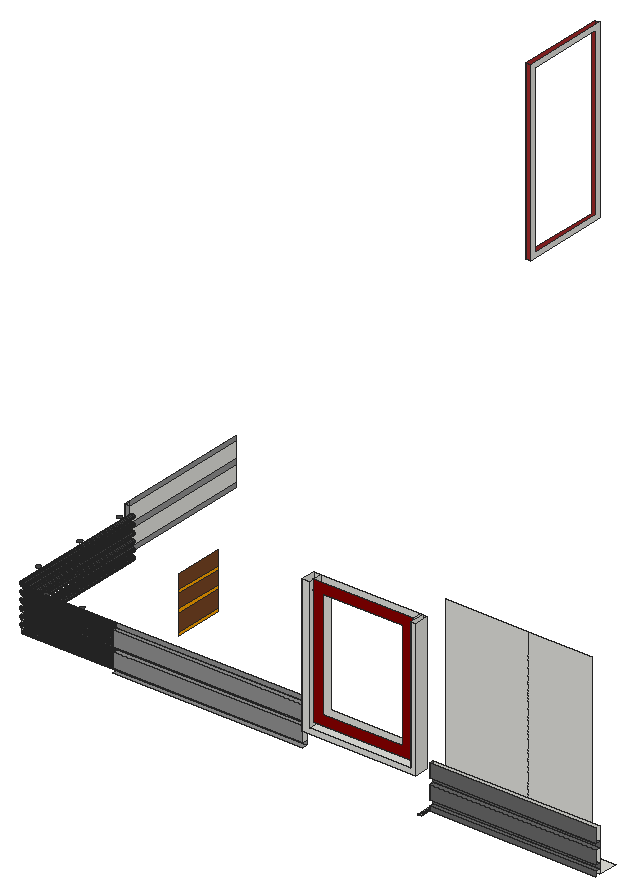
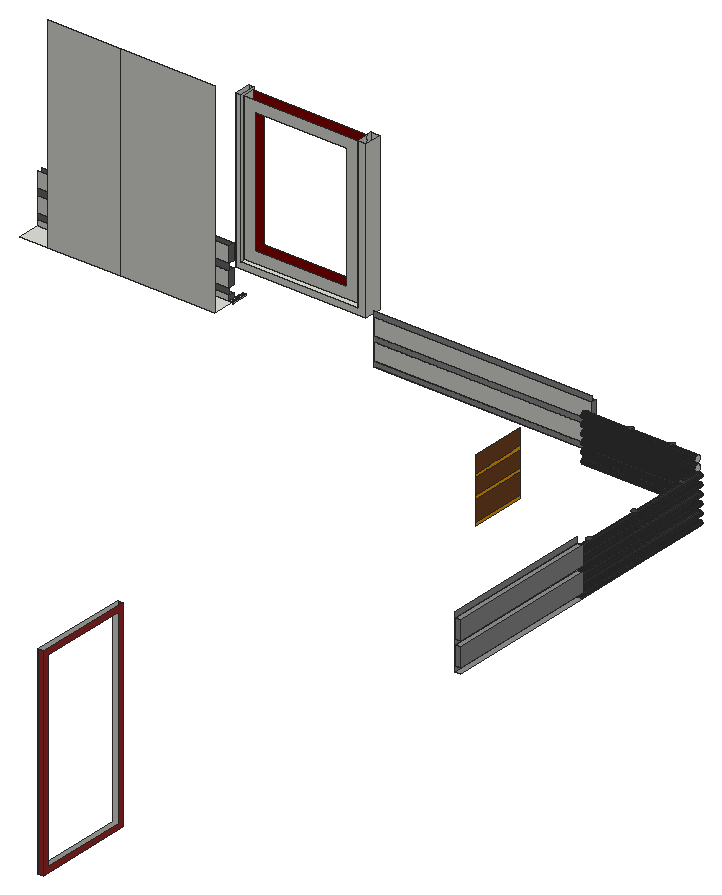
# SketchUp Ruby script. Lengths in inches.
U = 1.inch
M = Sketchup.active_model
def pt(a) = Geom::Point3d.new(a.map { |v| v * U })
def face(e, loops, mat)
  f = e.add_face(loops[0].map { |a| pt(a) })
  loops[1..].each { |l| e.add_face(l.map { |a| pt(a) }).erase! }
  f.material = f.back_material = mat if mat
  f
end
# faces: each face lists its corners as indices into pts; further lists are holes
def faces(e, pts, list, mat = nil) = list.each { |f| face(e, (f[0].is_a?(Array) ? f : [f]).map { |l| l.map { |i| pts[i] } }, mat) }
# xy, xz, yz: faces in a plane at the given z, y or x. An outline is a flat list of corners, or four numbers for a rectangle; further outlines are holes
def ring(l) = l.size == 4 ? [[l[0], l[1]], [l[2], l[1]], [l[2], l[3]], [l[0], l[3]]] : l.each_slice(2).to_a
def flat(e, list, mat, &to3) = list.each { |f| face(e, (f[0].is_a?(Array) ? f : [f]).map { |l| ring(l).map { |u, v| to3.(u, v) } }, mat) }
def xy(e, z, list, mat = nil) = flat(e, list, mat) { |x, y| [x, y, z] }
def xz(e, y, list, mat = nil) = flat(e, list, mat) { |x, z| [x, y, z] }
def yz(e, x, list, mat = nil) = flat(e, list, mat) { |y, z| [x, y, z] }
def lines(e, pts, list) = list.each { |a, b| e.add_line(pt(pts[a]), pt(pts[b])) }
# prism: a flat outline (further loops are holes) pulled along v
def prism(e, loops, v, mat = nil)
  f = face(e, loops, mat); d = Geom::Vector3d.new(v.map { |x| x * U })
  f.pushpull(f.normal.samedirection?(d) ? d.length : -d.length)
end
def box(e, o, s, mat = nil) = prism(e, [[o, [o[0] + s[0], o[1], o[2]], [o[0] + s[0], o[1] + s[1], o[2]], [o[0], o[1] + s[1], o[2]]]], [0, 0, s[2]], mat)
def at(x, y, z, deg = 0) = Geom::Transformation.translation(pt([x, y, z])) * Geom::Transformation.rotation(ORIGIN, Z_AXIS, deg.degrees)
def axes(o, x, y, z) = Geom::Transformation.new([*x, 0, *y, 0, *z, 0, *pt(o).to_a, 1])
def part(name) = M.definitions.add(name)
# library, detail: a bought-in or finely detailed component or shape, given as its bounding box
def library(name, o, s) = part(name).tap { |d| box(d.entities, o, s) }
def detail(e, o, s) = box(e.add_group.entities, o, s)
def put(e, d, t, mat = nil) = e.add_instance(d, t).tap { |i| i.material = mat if mat }
def group(e, t, mat = nil) = e.add_group.tap { |g| g.transformation = t; g.material = mat if mat }.entities
root = M.entities
M.materials.add("[0018_Brown]").color = [165, 42, 42]
M.materials.add("[0021_DarkRed]").color = [139, 0, 0]
M.materials.add("[0038_Orange]").color = [255, 165, 0]
M.materials.add("[0134_DimGray]").color = [105, 105, 105]
M.materials.add("[0137_Black]").color = [71, 71, 71]
M.materials.add("[Color M05]").color = [145, 145, 145]
M.materials.add("[Wood Veneer 01]").color = [120, 70, 37]
xy(root,247.03,[[8.875,116.75,11.875,199.5]],"[Color M05]")
xy(root,247.33,[[284.05,1.5,284.41,10.0625]])
xy(root,247.83,[[285.29,2.8125,286.17,10.0625]])
xy(root,247.89,[[284.05,1.0625,284.41,1.5],[284.41,1.0625,285.29,1.5625],[285.29,1.0625,286.17,2.8125],[284.05,1.5,284.41,10.0625],[284.41,1.5625,285.29,10.0625],
  [285.29,2.8125,286.17,10.0625],[286.17,7.0625,335.53,10.0625],[335.53,7.0625,375.29,10.0625],[284.41,10.0625,335.53,22.0625],[335.53,10.0625,390.0625,22.0625]])
xy(root,249.65,[[82.85,15.1875,200.79,18.1875]],"[Color M05]")
xy(root,250.07,[[8.875,116.75,11.875,199.5]],"[Color M05]")
xy(root,250.6875,[[286.17,7.0625,335.53,10.0625],[335.53,7.0625,390.0625,10.0625]],"[0134_DimGray]")
xy(root,252.55,[[82.85,15.1875,200.79,18.1875]])
xy(root,254.27,[[286.17,7.0625,390.0625,10.0625]],"[0134_DimGray]")
xy(root,260.15,[[8.875,116.75,11.875,199.5]],"[Color M05]")
xy(root,261.65,[[82.85,15.1875,200.79,18.1875]],"[Color M05]")
xy(root,262.6875,[[286.17,7.0625,390.0625,10.0625]],"[0134_DimGray]")
xy(root,263.19,[[8.875,116.75,11.875,199.5]],"[Color M05]")
xy(root,264.55,[[82.85,15.1875,200.79,18.1875]])
xy(root,266.27,[[286.17,7.0625,390.0625,10.0625]],"[0134_DimGray]")
xy(root,267.29,[[209.95,3.1875,280.75,12.1875]])
xy(root,270.55,[[214.5625,3.1875,278.01,12.1875]])
xy(root,271.42,[[12.37,43.72,12.71,43.74,13.04,43.84,13.33,44.02,13.56,44.27,13.72,44.58,13.79,44.91,13.78,45.25,13.68,45.58,13.49,45.87,13.24,46.1,12.9375,46.26,12.61,46.34,12.26,46.32,11.9375,46.22,11.65,46.04,11.41,45.79,11.25,45.48,11.18,45.15,11.19,44.81,11.29,44.48,11.48,44.1875,11.73,43.96,12.03,43.8],[12.37,75.91,12.71,75.92,13.04,76.03,13.33,76.21,13.56,76.46,13.72,76.76,13.79,77.1,13.78,77.44,13.68,77.77,13.49,78.06,13.24,78.29,12.9375,78.45,12.61,78.52,12.26,78.51,11.9375,78.41,11.65,78.23,11.41,77.97,11.25,77.67,11.18,77.34,11.19,76.99,11.29,76.67,11.48,76.375,11.73,76.14,12.03,75.99],[12.37,106.53,12.71,106.55,13.04,106.65,13.33,106.83,13.56,107.09,13.72,107.39,13.79,107.72,13.78,108.07,13.68,108.39,13.49,108.68,13.24,108.91,12.9375,109.07,12.61,109.15,12.26,109.14,11.9375,109.03,11.65,108.85,11.41,108.6,11.25,108.3,11.18,107.96,11.19,107.62,11.29,107.29,11.48,107,11.73,106.77,12.03,106.61]],"[0137_Black]")
xy(root,272.86,[[214.5625,6.1875,276.625,12.1875]])
xy(root,272.92,[[34.4,22.66,34.7,22.71,34.99,22.82,35.24,23.01,35.43,23.26,35.54,23.54,35.58,23.85,35.54,24.16,35.43,24.45,35.24,24.69,34.99,24.88,34.7,25,34.4,25.04,34.09,25,33.8,24.88,33.56,24.69,33.37,24.45,33.25,24.16,33.21,23.85,33.25,23.54,33.37,23.26,33.56,23.01,33.8,22.82,34.09,22.71],[56.47,23.05,56.78,23.09,57.0625,23.21,57.31,23.39,57.5,23.64,57.61,23.93,57.66,24.23,57.61,24.54,57.5,24.83,57.31,25.07,57.0625,25.26,56.78,25.38,56.47,25.42,56.16,25.38,55.875,25.26,55.63,25.07,55.44,24.83,55.32,24.54,55.28,24.23,55.32,23.93,55.44,23.64,55.63,23.39,55.875,23.21,56.16,23.09]],"[0137_Black]")
xy(root,273.08,[[8.875,428.78,11.875,482.72]],"[0018_Brown]")
xy(root,273.28,[[8.875,116.75,11.875,199.5]],"[Color M05]")
xy(root,273.65,[[82.85,15.1875,200.79,18.1875]],"[Color M05]")
xz(root,1.5,[[284.05,247.33,284.41,247.58],[284.05,247.58,284.41,247.89]])
xz(root,1.5625,[[284.41,247.7,285.29,247.89]])
xz(root,2.8125,[[285.29,247.64,286.17,247.83],[285.29,247.83,286.17,247.89]])
xz(root,3.1875,[[209.95,267.29,280.75,267.29,280.75,352.16,278.01,352.16,278.01,270.55,214.5625,270.55,214.5625,352.16,209.95,352.16]])
xz(root,6.1875,[[[214.5625,272.86,276.625,352.36],[220.5625,278.86,270.625,346.36]]],"[0021_DarkRed]")
xz(root,7.0625,[[286.17,247.89,390.0625,250.6875],[286.17,254.27,390.0625,262.6875],[286.17,266.27,390.0625,274.6875]],"[0134_DimGray]")
xz(root,10.0625,[[284.05,247.33,284.41,247.89],[285.29,247.83,286.17,247.89],[286.17,247.89,390.0625,250.6875],[286.17,254.27,390.0625,262.6875],[286.17,266.27,390.0625,274.6875]])
xz(root,10.0625,[[286.17,250.6875,390.0625,254.27],[286.17,262.6875,390.0625,266.27]],"[0134_DimGray]")
xz(root,12.1875,[[209.95,267.29,280.75,267.29,280.75,352.16,278.01,352.16,278.01,270.55,214.5625,270.55,214.5625,352.16,209.95,352.16],[[214.5625,272.86,276.625,352.16],[220.5625,278.86,270.625,346.36]]])
xz(root,15.1875,[[82.85,252.55,200.79,261.65],[82.85,264.55,200.79,273.65]],"[Color M05]")
xz(root,18.1875,[[82.85,252.55,200.79,261.65],[82.85,264.55,200.79,273.65]])
xz(root,18.1875,[[82.85,249.65,200.79,252.55],[82.85,261.65,200.79,264.55],[82.85,273.65,200.79,276.55]],"[Color M05]")
xz(root,22.0625,[[284.41,247.89,335.53,358.6875],[335.53,247.89,375.29,358.6875]])
xz(root,116.75,[[8.875,250.07,11.875,260.15]],"[0134_DimGray]")
xz(root,116.75,[[8.875,263.19,11.875,273.28]],"[Color M05]")
xz(root,199.5,[[8.875,250.07,11.875,260.15],[8.875,263.19,11.875,273.28]],"[Color M05]")
xz(root,428.78,[[8.875,273.08,11.875,382.4]],"[0018_Brown]")
xz(root,482.72,[[8.875,273.08,11.875,382.4]],"[0018_Brown]")
yz(root,8.875,[[[428.78,273.08,482.72,382.4],[431.78,276.08,479.72,379.4]]],"[0018_Brown]")
yz(root,8.875,[[116.75,250.07,199.5,260.15],[116.75,263.19,199.5,273.28]],"[Color M05]")
yz(root,11.875,[[116.75,250.07,199.5,260.15],[116.75,263.19,199.5,273.28],[[428.78,273.08,482.72,382.4],[431.78,276.08,479.72,379.4]]])
yz(root,11.875,[[116.75,247.03,199.5,250.07],[116.75,260.15,199.5,263.19],[116.75,273.28,199.5,276.32]],"[Color M05]")
yz(root,20.6875,[[23.69,246.4,24.13,246.46,24.54,246.625,24.89,246.89,25.15,247.24,25.32,247.65,25.38,248.09,25.32,248.52,25.15,248.93,24.89,249.28,24.54,249.55,24.13,249.72,23.69,249.78,23.26,249.72,22.85,249.55,22.5,249.28,22.23,248.93,22.0625,248.52,22.0625,247.65,22.23,247.24,22.5,246.89,22.85,246.625,23.26,246.46],[23.69,250.84,24.13,250.9,24.54,251.0625,24.89,251.33,25.15,251.68,25.32,252.09,25.38,252.53,25.32,252.96,25.15,253.37,24.89,253.72,24.54,253.99,24.13,254.16,23.69,254.21,23.26,254.16,22.85,253.99,22.5,253.72,22.23,253.37,22.0625,252.96,22.0625,252.09,22.23,251.68,22.5,251.33,22.85,251.0625,23.26,250.9],[23.69,255.28,24.13,255.33,24.54,255.5,24.89,255.77,25.15,256.12,25.32,256.53,25.38,256.96,25.32,257.4,25.15,257.81,24.89,258.16,24.54,258.42,24.13,258.59,23.69,258.65,23.26,258.59,22.85,258.42,22.5,258.16,22.23,257.81,22.0625,257.4,22.0625,256.53,22.23,256.12,22.5,255.77,22.85,255.5,23.26,255.33],[23.69,259.71,24.13,259.77,24.54,259.9375,24.89,260.21,25.15,260.56,25.32,260.96,25.38,261.4,25.32,261.84,25.15,262.24,24.89,262.59,24.54,262.86,24.13,263.03,23.69,263.09,23.26,263.03,22.85,262.86,22.5,262.59,22.23,262.24,22.0625,261.84,22.0625,260.96,22.23,260.56,22.5,260.21,22.85,259.9375,23.26,259.77],[23.69,264.15,24.13,264.21,24.54,264.375,24.89,264.64,25.15,264.99,25.32,265.4,25.38,265.84,25.32,266.27,25.15,266.68,24.89,267.03,24.54,267.3,24.13,267.47,23.69,267.53,23.26,267.47,22.85,267.3,22.5,267.03,22.23,266.68,22.0625,266.27,22.0625,265.4,22.23,264.99,22.5,264.64,22.85,264.375,23.26,264.21],
  [23.69,268.59,24.13,268.65,24.54,268.8125,24.89,269.08,25.15,269.43,25.32,269.84,25.38,270.28,25.32,270.71,25.15,271.12,24.89,271.47,24.54,271.74,24.13,271.91,23.69,271.96,23.26,271.91,22.85,271.74,22.5,271.47,22.23,271.12,22.0625,270.71,22.0625,269.84,22.23,269.43,22.5,269.08,22.85,268.8125,23.26,268.65]])
yz(root,82.85,[[66.65,247.86,96.65,249.57],[66.65,260.99,96.65,262.69],[66.65,271.74,96.65,273.44]],"[0038_Orange]")
yz(root,82.85,[[15.1875,252.55,18.1875,261.65],[15.1875,264.55,18.1875,273.65]],"[Color M05]")
yz(root,82.85,[[66.65,249.57,96.65,260.99],[66.65,262.69,96.65,271.74],[66.65,273.44,96.65,282.49]],"[Wood Veneer 01]")
yz(root,200.79,[[15.1875,252.55,18.1875,261.65],[15.1875,264.55,18.1875,273.65]])
yz(root,209.95,[[3.1875,267.29,12.1875,352.16]])
yz(root,214.5625,[[3.1875,270.55,12.1875,270.55,12.1875,272.86,6.1875,272.86,6.1875,352.16,3.1875,352.16],[6.1875,272.86,12.1875,352.16]])
yz(root,276.625,[[6.1875,272.86,12.1875,352.16]])
yz(root,278.01,[[3.1875,270.55,12.1875,352.16]])
yz(root,280.75,[[3.1875,267.29,12.1875,352.16]])
yz(root,284.05,[[1.5,247.33,10.0625,247.89],[1.0625,247.58,1.5,247.89]])
yz(root,284.41,[[1.5,247.33,1.5625,247.7],[1.5625,247.33,10.0625,247.89],[1.5,247.7,1.5625,247.89]])
yz(root,285.29,[[1.5625,247.64,2.8125,247.89],[2.8125,247.83,10.0625,247.89]])
yz(root,286.17,[[2.8125,247.83,10.0625,247.89]])
yz(root,286.17,[[7.0625,247.89,10.0625,250.6875],[7.0625,254.27,10.0625,262.6875],[7.0625,266.27,10.0625,274.6875]],"[0134_DimGray]")
p = [[13.62,31.0625,243.74],[13.26,31.0625,243.79],[13.26,116.75,243.79],[13.62,116.75,243.74],[13.97,31.0625,243.79],[13.97,116.75,243.79],
  [12.93,31.0625,243.93],[12.93,116.75,243.93],[14.31,31.0625,243.93],[14.31,116.75,243.93],[12.65,31.0625,244.15],[12.65,116.75,244.15],
  [14.59,31.0625,244.15],[14.59,116.75,244.15],[12.43,31.0625,244.43],[12.43,116.75,244.43],[14.81,31.0625,244.43],[14.81,116.75,244.43],
  [12.29,31.0625,244.76],[12.29,116.75,244.76],[14.95,31.0625,244.76],[14.95,116.75,244.76],[12.24,31.0625,245.12],[12.24,116.75,245.12],
  [14.99,31.0625,245.12],[14.99,116.75,245.12],[12.29,31.0625,245.47],[12.29,116.75,245.47],[14.95,31.0625,245.47],[14.95,116.75,245.47],
  [12.43,31.0625,245.81],[12.43,116.75,245.81],[14.81,31.0625,245.81],[14.81,116.75,245.81],[12.65,31.0625,246.09],[12.65,116.75,246.09],
  [14.59,31.0625,246.09],[14.59,116.75,246.09],[12.93,31.0625,246.31],[12.93,116.75,246.31],[14.31,31.0625,246.31],[14.31,116.75,246.31],
  [13.26,31.0625,246.45],[13.26,116.75,246.45],[13.97,31.0625,246.45],[13.97,116.75,246.45],[20.6875,23.26,246.46],[20.6875,23.69,246.4],
  [82.66,23.69,246.4],[82.66,23.26,246.46],[20.6875,24.13,246.46],[82.66,24.13,246.46],[13.62,31.0625,246.49],[13.62,116.75,246.49],
  [20.6875,22.85,246.625],[82.66,22.85,246.625],[20.6875,24.54,246.625],[82.66,24.54,246.625],[20.6875,22.5,246.89],[82.66,22.5,246.89],
  [20.6875,24.89,246.89],[82.66,24.89,246.89],[20.6875,22.23,247.24],[82.66,22.23,247.24],[20.6875,25.15,247.24],[82.66,25.15,247.24],
  [20.6875,22.0625,247.65],[82.66,22.0625,247.65],[20.6875,25.32,247.65],[82.66,25.32,247.65],[20.6875,22,248.09],[82.66,22,248.09],
  [20.6875,25.38,248.09],[82.66,25.38,248.09],[20.6875,22.0625,248.52],[82.66,22.0625,248.52],[20.6875,25.32,248.52],[82.66,25.32,248.52],
  [13.26,31.0625,248.41],[12.93,31.0625,248.55],[12.93,116.75,248.55],[13.26,116.75,248.41],[13.62,31.0625,248.37],[13.62,116.75,248.37],
  [13.97,31.0625,248.41],[13.97,116.75,248.41],[14.31,31.0625,248.55],[14.31,116.75,248.55],[20.6875,22.23,248.93],[82.66,22.23,248.93],
  [20.6875,25.15,248.93],[82.66,25.15,248.93],[12.65,31.0625,248.77],[12.65,116.75,248.77],[14.59,31.0625,248.77],[14.59,116.75,248.77],
  [12.43,31.0625,249.06],[12.43,116.75,249.06],[14.81,31.0625,249.06],[14.81,116.75,249.06],[20.6875,22.5,249.28],[82.66,22.5,249.28],
  [20.6875,24.89,249.28],[82.66,24.89,249.28],[12.29,31.0625,249.39],[12.29,116.75,249.39],[14.95,31.0625,249.39],[14.95,116.75,249.39],
  [20.6875,22.85,249.55],[82.66,22.85,249.55],[20.6875,24.54,249.55],[82.66,24.54,249.55],[12.24,31.0625,249.74],[12.24,116.75,249.74],
  [14.99,31.0625,249.74],[14.99,116.75,249.74],[20.6875,23.26,249.72],[82.66,23.26,249.72],[20.6875,24.13,249.72],[82.66,24.13,249.72],
  [20.6875,23.69,249.78],[82.66,23.69,249.78],[12.29,31.0625,250.1],[12.29,116.75,250.1],[14.95,31.0625,250.1],[14.95,116.75,250.1],
  [12.43,31.0625,250.43],[12.43,116.75,250.43],[14.81,31.0625,250.43],[14.81,116.75,250.43],[12.65,31.0625,250.71],[12.65,116.75,250.71],
  [14.59,31.0625,250.71],[14.59,116.75,250.71],[12.93,31.0625,250.93],[12.93,116.75,250.93],[14.31,31.0625,250.93],[14.31,116.75,250.93],
  [20.6875,23.26,250.9],[20.6875,23.69,250.84],[82.66,23.69,250.84],[82.66,23.26,250.9],[20.6875,24.13,250.9],[82.66,24.13,250.9],
  [20.6875,22.85,251.0625],[82.66,22.85,251.0625],[20.6875,24.54,251.0625],[82.66,24.54,251.0625],[13.26,31.0625,251.07],[13.26,116.75,251.07],
  [13.97,31.0625,251.07],[13.97,116.75,251.07],[20.6875,22.5,251.33],[82.66,22.5,251.33],[20.6875,24.89,251.33],[82.66,24.89,251.33],
  [13.62,31.0625,251.12],[13.62,116.75,251.12],[20.6875,22.23,251.68],[82.66,22.23,251.68],[20.6875,25.15,251.68],[82.66,25.15,251.68],
  [20.6875,22.0625,252.09],[82.66,22.0625,252.09],[20.6875,25.32,252.09],[82.66,25.32,252.09],[20.6875,22,252.53],[82.66,22,252.53],
  [20.6875,25.38,252.53],[82.66,25.38,252.53],[20.6875,22.0625,252.96],[82.66,22.0625,252.96],[20.6875,25.32,252.96],[82.66,25.32,252.96],
  [20.6875,22.23,253.37],[82.66,22.23,253.37],[20.6875,25.15,253.37],[82.66,25.15,253.37],[13.26,31.0625,253.04],[12.93,31.0625,253.18],
  [12.93,116.75,253.18],[13.26,116.75,253.04],[13.62,31.0625,252.99],[13.62,116.75,252.99],[13.97,31.0625,253.04],[13.97,116.75,253.04],
  [14.31,31.0625,253.18],[14.31,116.75,253.18],[12.65,31.0625,253.4],[12.65,116.75,253.4],[14.59,31.0625,253.4],[14.59,116.75,253.4],
  [20.6875,22.5,253.72],[82.66,22.5,253.72],[20.6875,24.89,253.72],[82.66,24.89,253.72],[12.43,31.0625,253.68],[12.43,116.75,253.68],
  [14.81,31.0625,253.68],[14.81,116.75,253.68],[20.6875,22.85,253.99],[82.66,22.85,253.99],[20.6875,24.54,253.99],[82.66,24.54,253.99],
  [12.29,31.0625,254.01],[12.29,116.75,254.01],[14.95,31.0625,254.01],[14.95,116.75,254.01],[20.6875,23.26,254.16],[82.66,23.26,254.16],
  [20.6875,24.13,254.16],[82.66,24.13,254.16],[12.24,31.0625,254.37],[12.24,116.75,254.37],[14.99,31.0625,254.37],[14.99,116.75,254.37],
  [20.6875,23.69,254.21],[82.66,23.69,254.21],[12.29,31.0625,254.72],[12.29,116.75,254.72],[14.95,31.0625,254.72],[14.95,116.75,254.72],
  [12.43,31.0625,255.06],[12.43,116.75,255.06],[14.81,31.0625,255.06],[14.81,116.75,255.06],[12.65,31.0625,255.34],[12.65,116.75,255.34],
  [14.59,31.0625,255.34],[14.59,116.75,255.34],[20.6875,22.85,255.5],[20.6875,23.26,255.33],[82.66,23.26,255.33],[82.66,22.85,255.5],
  [20.6875,23.69,255.28],[82.66,23.69,255.28],[20.6875,24.13,255.33],[82.66,24.13,255.33],[20.6875,24.54,255.5],[82.66,24.54,255.5],
  [12.93,31.0625,255.56],[12.93,116.75,255.56],[14.31,31.0625,255.56],[14.31,116.75,255.56],[20.6875,22.5,255.77],[82.66,22.5,255.77],
  [20.6875,24.89,255.77],[82.66,24.89,255.77],[13.26,31.0625,255.7],[13.26,116.75,255.7],[13.97,31.0625,255.7],[13.97,116.75,255.7],
  [13.62,31.0625,255.74],[13.62,116.75,255.74],[20.6875,22.23,256.12],[82.66,22.23,256.12],[20.6875,25.15,256.12],[82.66,25.15,256.12],
  [20.6875,22.0625,256.53],[82.66,22.0625,256.53],[20.6875,25.32,256.53],[82.66,25.32,256.53],[20.6875,22,256.96],[82.66,22,256.96],
  [20.6875,25.38,256.96],[82.66,25.38,256.96],[20.6875,22.0625,257.4],[82.66,22.0625,257.4],[20.6875,25.32,257.4],[82.66,25.32,257.4],
  [20.6875,22.23,257.81],[82.66,22.23,257.81],[20.6875,25.15,257.81],[82.66,25.15,257.81],[13.62,31.0625,257.62],[13.26,31.0625,257.66],
  [13.26,116.75,257.66],[13.62,116.75,257.62],[13.97,31.0625,257.66],[13.97,116.75,257.66],[12.93,31.0625,257.8],[12.93,116.75,257.8],
  [14.31,31.0625,257.8],[14.31,116.75,257.8],[20.6875,22.5,258.16],[82.66,22.5,258.16],[20.6875,24.89,258.16],[82.66,24.89,258.16],
  [12.65,31.0625,258.02],[12.65,116.75,258.02],[14.59,31.0625,258.02],[14.59,116.75,258.02],[12.43,31.0625,258.31],[12.43,116.75,258.31],
  [14.81,31.0625,258.31],[14.81,116.75,258.31],[20.6875,22.85,258.42],[82.66,22.85,258.42],[20.6875,24.54,258.42],[82.66,24.54,258.42],
  [12.29,31.0625,258.64],[12.29,116.75,258.64],[14.95,31.0625,258.64],[14.95,116.75,258.64],[20.6875,23.26,258.59],[82.66,23.26,258.59],
  [20.6875,24.13,258.59],[82.66,24.13,258.59],[20.6875,23.69,258.65],[82.66,23.69,258.65],[12.24,31.0625,258.99],[12.24,116.75,258.99],
  [14.99,31.0625,258.99],[14.99,116.75,258.99],[12.29,31.0625,259.35],[12.29,116.75,259.35],[14.95,31.0625,259.35],[14.95,116.75,259.35],
  [12.43,31.0625,259.68],[12.43,116.75,259.68],[14.81,31.0625,259.68],[14.81,116.75,259.68],[20.6875,23.26,259.77],[20.6875,23.69,259.71],
  [82.66,23.69,259.71],[82.66,23.26,259.77],[20.6875,24.13,259.77],[82.66,24.13,259.77],[12.65,31.0625,259.96],[12.65,116.75,259.96],
  [14.59,31.0625,259.96],[14.59,116.75,259.96],[20.6875,22.85,259.9375],[82.66,22.85,259.9375],[20.6875,24.54,259.9375],[82.66,24.54,259.9375],
  [20.6875,22.5,260.21],[82.66,22.5,260.21],[20.6875,24.89,260.21],[82.66,24.89,260.21],[12.93,31.0625,260.18],[12.93,116.75,260.18],
  [14.31,31.0625,260.18],[14.31,116.75,260.18],[20.6875,22.23,260.56],[82.66,22.23,260.56],[20.6875,25.15,260.56],[82.66,25.15,260.56],
  [13.26,31.0625,260.32],[13.26,116.75,260.32],[13.97,31.0625,260.32],[13.97,116.75,260.32],[13.62,31.0625,260.37],[13.62,116.75,260.37],
  [20.6875,22.0625,260.96],[82.66,22.0625,260.96],[20.6875,25.32,260.96],[82.66,25.32,260.96],[20.6875,22,261.4],[82.66,22,261.4],
  [20.6875,25.38,261.4],[82.66,25.38,261.4],[20.6875,22.0625,261.84],[82.66,22.0625,261.84],[20.6875,25.32,261.84],[82.66,25.32,261.84],
  [20.6875,22.23,262.24],[82.66,22.23,262.24],[20.6875,25.15,262.24],[82.66,25.15,262.24],[20.6875,22.5,262.59],[82.66,22.5,262.59],
  [20.6875,24.89,262.59],[82.66,24.89,262.59],[13.62,31.0625,262.24],[13.26,31.0625,262.29],[13.26,116.75,262.29],[13.62,116.75,262.24],
  [13.97,31.0625,262.29],[13.97,116.75,262.29],[12.93,31.0625,262.43],[12.93,116.75,262.43],[14.31,31.0625,262.43],[14.31,116.75,262.43],
  [12.65,31.0625,262.65],[12.65,116.75,262.65],[14.59,31.0625,262.65],[14.59,116.75,262.65],[20.6875,22.85,262.86],[82.66,22.85,262.86],
  [20.6875,24.54,262.86],[82.66,24.54,262.86],[12.43,31.0625,262.93],[12.43,116.75,262.93],[14.81,31.0625,262.93],[14.81,116.75,262.93],
  [20.6875,23.26,263.03],[82.66,23.26,263.03],[20.6875,24.13,263.03],[82.66,24.13,263.03],[12.29,31.0625,263.26],[12.29,116.75,263.26],
  [14.95,31.0625,263.26],[14.95,116.75,263.26],[20.6875,23.69,263.09],[82.66,23.69,263.09],[12.24,31.0625,263.62],[12.24,116.75,263.62],
  [14.99,31.0625,263.62],[14.99,116.75,263.62],[12.29,31.0625,263.97],[12.29,116.75,263.97],[14.95,31.0625,263.97],[14.95,116.75,263.97],
  [12.43,31.0625,264.31],[12.43,116.75,264.31],[14.81,31.0625,264.31],[14.81,116.75,264.31],[20.6875,22.85,264.375],[20.6875,23.26,264.21],
  [82.66,23.26,264.21],[82.66,22.85,264.375],[20.6875,23.69,264.15],[82.66,23.69,264.15],[20.6875,24.13,264.21],[82.66,24.13,264.21],
  [20.6875,24.54,264.375],[82.66,24.54,264.375],[12.65,31.0625,264.59],[12.65,116.75,264.59],[14.59,31.0625,264.59],[14.59,116.75,264.59],
  [20.6875,22.5,264.64],[82.66,22.5,264.64],[20.6875,24.89,264.64],[82.66,24.89,264.64],[20.6875,22.23,264.99],[82.66,22.23,264.99],
  [20.6875,25.15,264.99],[82.66,25.15,264.99],[12.93,31.0625,264.81],[12.93,116.75,264.81],[14.31,31.0625,264.81],[14.31,116.75,264.81],
  [13.26,31.0625,264.95],[13.26,116.75,264.95],[13.97,31.0625,264.95],[13.97,116.75,264.95],[13.62,31.0625,264.99],[13.62,116.75,264.99],
  [20.6875,22.0625,265.4],[82.66,22.0625,265.4],[20.6875,25.32,265.4],[82.66,25.32,265.4],[20.6875,22,265.84],[82.66,22,265.84],
  [20.6875,25.38,265.84],[82.66,25.38,265.84],[20.6875,22.0625,266.27],[82.66,22.0625,266.27],[20.6875,25.32,266.27],[82.66,25.32,266.27],
  [20.6875,22.23,266.68],[82.66,22.23,266.68],[20.6875,25.15,266.68],[82.66,25.15,266.68],[20.6875,22.5,267.03],[82.66,22.5,267.03],
  [20.6875,24.89,267.03],[82.66,24.89,267.03],[13.26,31.0625,266.91],[12.93,31.0625,267.05],[12.93,116.75,267.05],[13.26,116.75,266.91],
  [13.62,31.0625,266.87],[13.62,116.75,266.87],[13.97,31.0625,266.91],[13.97,116.75,266.91],[14.31,31.0625,267.05],[14.31,116.75,267.05],
  [20.6875,22.85,267.3],[82.66,22.85,267.3],[20.6875,24.54,267.3],[82.66,24.54,267.3],[12.65,31.0625,267.27],[12.65,116.75,267.27],
  [14.59,31.0625,267.27],[14.59,116.75,267.27],[20.6875,23.26,267.47],[82.66,23.26,267.47],[20.6875,24.13,267.47],[82.66,24.13,267.47],
  [12.43,31.0625,267.56],[12.43,116.75,267.56],[14.81,31.0625,267.56],[14.81,116.75,267.56],[20.6875,23.69,267.53],[82.66,23.69,267.53],
  [12.29,31.0625,267.89],[12.29,116.75,267.89],[14.95,31.0625,267.89],[14.95,116.75,267.89],[12.24,31.0625,268.24],[12.24,116.75,268.24],
  [14.99,31.0625,268.24],[14.99,116.75,268.24],[12.29,31.0625,268.6],[12.29,116.75,268.6],[14.95,31.0625,268.6],[14.95,116.75,268.6],
  [20.6875,22.85,268.8125],[20.6875,23.26,268.65],[82.66,23.26,268.65],[82.66,22.85,268.8125],[20.6875,23.69,268.59],[82.66,23.69,268.59],
  [20.6875,24.13,268.65],[82.66,24.13,268.65],[20.6875,24.54,268.8125],[82.66,24.54,268.8125],[12.43,31.0625,268.93],[12.43,116.75,268.93],
  [14.81,31.0625,268.93],[14.81,116.75,268.93],[20.6875,22.5,269.08],[82.66,22.5,269.08],[20.6875,24.89,269.08],[82.66,24.89,269.08],
  [12.65,31.0625,269.21],[12.65,116.75,269.21],[14.59,31.0625,269.21],[14.59,116.75,269.21],[20.6875,22.23,269.43],[82.66,22.23,269.43],
  [20.6875,25.15,269.43],[82.66,25.15,269.43],[12.93,31.0625,269.43],[12.93,116.75,269.43],[14.31,31.0625,269.43],[14.31,116.75,269.43],
  [20.6875,22.0625,269.84],[82.66,22.0625,269.84],[20.6875,25.32,269.84],[82.66,25.32,269.84],[13.26,31.0625,269.57],[13.26,116.75,269.57],
  [13.97,31.0625,269.57],[13.97,116.75,269.57],[13.62,31.0625,269.62],[13.62,116.75,269.62],[20.6875,22,270.28],[82.66,22,270.28],
  [20.6875,25.38,270.28],[82.66,25.38,270.28],[20.6875,22.0625,270.71],[82.66,22.0625,270.71],[20.6875,25.32,270.71],[82.66,25.32,270.71],
  [20.6875,22.23,271.12],[82.66,22.23,271.12],[20.6875,25.15,271.12],[82.66,25.15,271.12],[20.6875,22.5,271.47],[82.66,22.5,271.47],
  [20.6875,24.89,271.47],[82.66,24.89,271.47],[20.6875,22.85,271.74],[82.66,22.85,271.74],[20.6875,24.54,271.74],[82.66,24.54,271.74],
  [20.6875,23.26,271.91],[82.66,23.26,271.91],[20.6875,24.13,271.91],[82.66,24.13,271.91],[20.6875,23.69,271.96],[82.66,23.69,271.96],
  [286.52,1.0625,244.84],[286.52,4.0625,244.84],[286.99,4.0625,244.84],[284.41,1.5,247.7],[284.41,1.0625,247.7],[286.17,2.8125,247.64],
  [286.17,1.0625,247.64],[284.41,1.5,247.58],[284.41,1.0625,247.58]]
faces(root,p,[[0,1,2,3],[4,0,3,5],[1,6,7,2],[8,4,5,9],[6,10,11,7],[12,8,9,13],[10,14,15,11],[16,12,13,17],
  [14,18,19,15],[20,16,17,21],[18,22,23,19],[24,20,21,25],[22,26,27,23],[28,24,25,29],[26,30,31,27],[32,28,29,33],
  [30,34,35,31],[36,32,33,37],[34,38,39,35],[40,36,37,41],[38,42,43,39],[44,40,41,45],[46,47,48,49],[47,50,51,48],
  [42,52,53,43],[52,44,45,53],[54,46,49,55],[50,56,57,51],[58,54,55,59],[56,60,61,57],[62,58,59,63],[60,64,65,61],
  [66,62,63,67],[64,68,69,65],[70,66,67,71],[68,72,73,69],[74,70,71,75],[72,76,77,73],[78,79,80,81],[82,78,81,83],
  [84,82,83,85],[86,84,85,87],[88,74,75,89],[76,90,91,77],[79,92,93,80],[94,86,87,95],[92,96,97,93],[98,94,95,99],
  [100,88,89,101],[90,102,103,91],[96,104,105,97],[106,98,99,107],[108,100,101,109],[102,110,111,103],[104,112,113,105],[114,106,107,115],
  [116,108,109,117],[110,118,119,111],[120,116,117,121],[118,120,121,119],[112,122,123,113],[124,114,115,125],[122,126,127,123],[128,124,125,129],
  [126,130,131,127],[132,128,129,133],[130,134,135,131],[136,132,133,137],[138,139,140,141],[139,142,143,140],[144,138,141,145],[142,146,147,143],
  [134,148,149,135],[150,136,137,151],[152,144,145,153],[146,154,155,147],[148,156,157,149],[156,150,151,157],[158,152,153,159],[154,160,161,155],
  [162,158,159,163],[160,164,165,161],[166,162,163,167],[164,168,169,165],[170,166,167,171],[168,172,173,169],[174,170,171,175],[172,176,177,173],
  [178,179,180,181],[182,178,181,183],[184,182,183,185],[186,184,185,187],[179,188,189,180],[190,186,187,191],[192,174,175,193],[176,194,195,177],
  [188,196,197,189],[198,190,191,199],[200,192,193,201],[194,202,203,195],[196,204,205,197],[206,198,199,207],[208,200,201,209],[202,210,211,203],
  [204,212,213,205],[214,206,207,215],[216,208,209,217],[210,216,217,211],[212,218,219,213],[220,214,215,221],[218,222,223,219],[224,220,221,225],
  [222,226,227,223],[228,224,225,229],[230,231,232,233],[231,234,235,232],[234,236,237,235],[236,238,239,237],[226,240,241,227],[242,228,229,243],
  [244,230,233,245],[238,246,247,239],[240,248,249,241],[250,242,243,251],[248,252,253,249],[252,250,251,253],[254,244,245,255],[246,256,257,247],
  [258,254,255,259],[256,260,261,257],[262,258,259,263],[260,264,265,261],[266,262,263,267],[264,268,269,265],[270,266,267,271],[268,272,273,269],
  [274,275,276,277],[278,274,277,279],[275,280,281,276],[282,278,279,283],[284,270,271,285],[272,286,287,273],[280,288,289,281],[290,282,283,291],
  [288,292,293,289],[294,290,291,295],[296,284,285,297],[286,298,299,287],[292,300,301,293],[302,294,295,303],[304,296,297,305],[298,306,307,299],
  [308,304,305,309],[306,308,309,307],[300,310,311,301],[312,302,303,313],[310,314,315,311],[316,312,313,317],[314,318,319,315],[320,316,317,321],
  [322,323,324,325],[323,326,327,324],[318,328,329,319],[330,320,321,331],[332,322,325,333],[326,334,335,327],[336,332,333,337],[334,338,339,335],
  [328,340,341,329],[342,330,331,343],[344,336,337,345],[338,346,347,339],[340,348,349,341],[350,342,343,351],[348,352,353,349],[352,350,351,353],
  [354,344,345,355],[346,356,357,347],[358,354,355,359],[356,360,361,357],[362,358,359,363],[360,364,365,361],[366,362,363,367],[364,368,369,365],
  [370,366,367,371],[368,372,373,369],[374,375,376,377],[378,374,377,379],[375,380,381,376],[382,378,379,383],[380,384,385,381],[386,382,383,387],
  [388,370,371,389],[372,390,391,373],[384,392,393,385],[394,386,387,395],[396,388,389,397],[390,398,399,391],[392,400,401,393],[402,394,395,403],
  [404,396,397,405],[398,404,405,399],[400,406,407,401],[408,402,403,409],[406,410,411,407],[412,408,409,413],[410,414,415,411],[416,412,413,417],
  [418,419,420,421],[419,422,423,420],[422,424,425,423],[424,426,427,425],[414,428,429,415],[430,416,417,431],[432,418,421,433],[426,434,435,427],
  [436,432,433,437],[434,438,439,435],[428,440,441,429],[442,430,431,443],[440,444,445,441],[446,442,443,447],[444,448,449,445],[448,446,447,449],
  [450,436,437,451],[438,452,453,439],[454,450,451,455],[452,456,457,453],[458,454,455,459],[456,460,461,457],[462,458,459,463],[460,464,465,461],
  [466,462,463,467],[464,468,469,465],[470,471,472,473],[474,470,473,475],[476,474,475,477],[478,476,477,479],[480,466,467,481],[468,482,483,469],
  [471,484,485,472],[486,478,479,487],[488,480,481,489],[482,490,491,483],[484,492,493,485],[494,486,487,495],[496,488,489,497],[490,496,497,491],
  [492,498,499,493],[500,494,495,501],[498,502,503,499],[504,500,501,505],[502,506,507,503],[508,504,505,509],[510,511,512,513],[511,514,515,512],
  [514,516,517,515],[516,518,519,517],[506,520,521,507],[522,508,509,523],[524,510,513,525],[518,526,527,519],[520,528,529,521],[530,522,523,531],
  [532,524,525,533],[526,534,535,527],[528,536,537,529],[538,530,531,539],[540,532,533,541],[534,542,543,535],[536,544,545,537],[546,538,539,547],
  [544,548,549,545],[548,546,547,549],[550,540,541,551],[542,552,553,543],[554,550,551,555],[552,556,557,553],[558,554,555,559],[556,560,561,557],
  [562,558,559,563],[560,564,565,561],[566,562,563,567],[564,568,569,565],[570,566,567,571],[568,572,573,569],[574,570,571,575],[572,574,575,573]],"[0137_Black]")
lines(root,p,[[576,577],[578,577],[579,580],[581,582],[583,584]])
